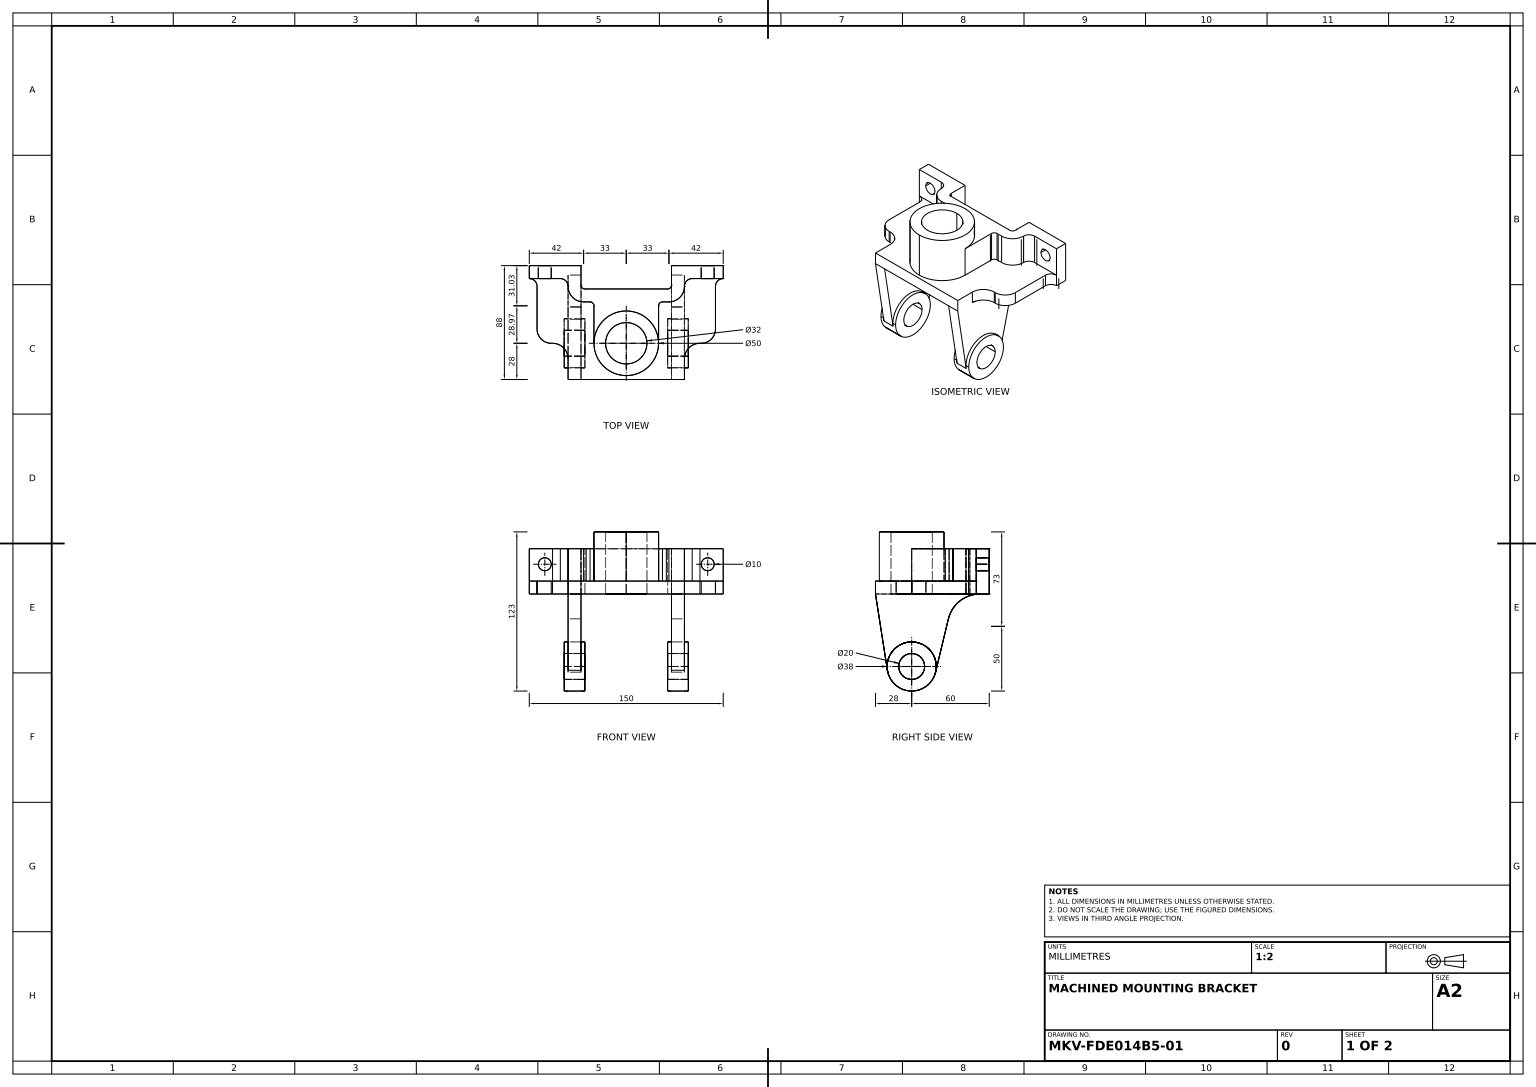
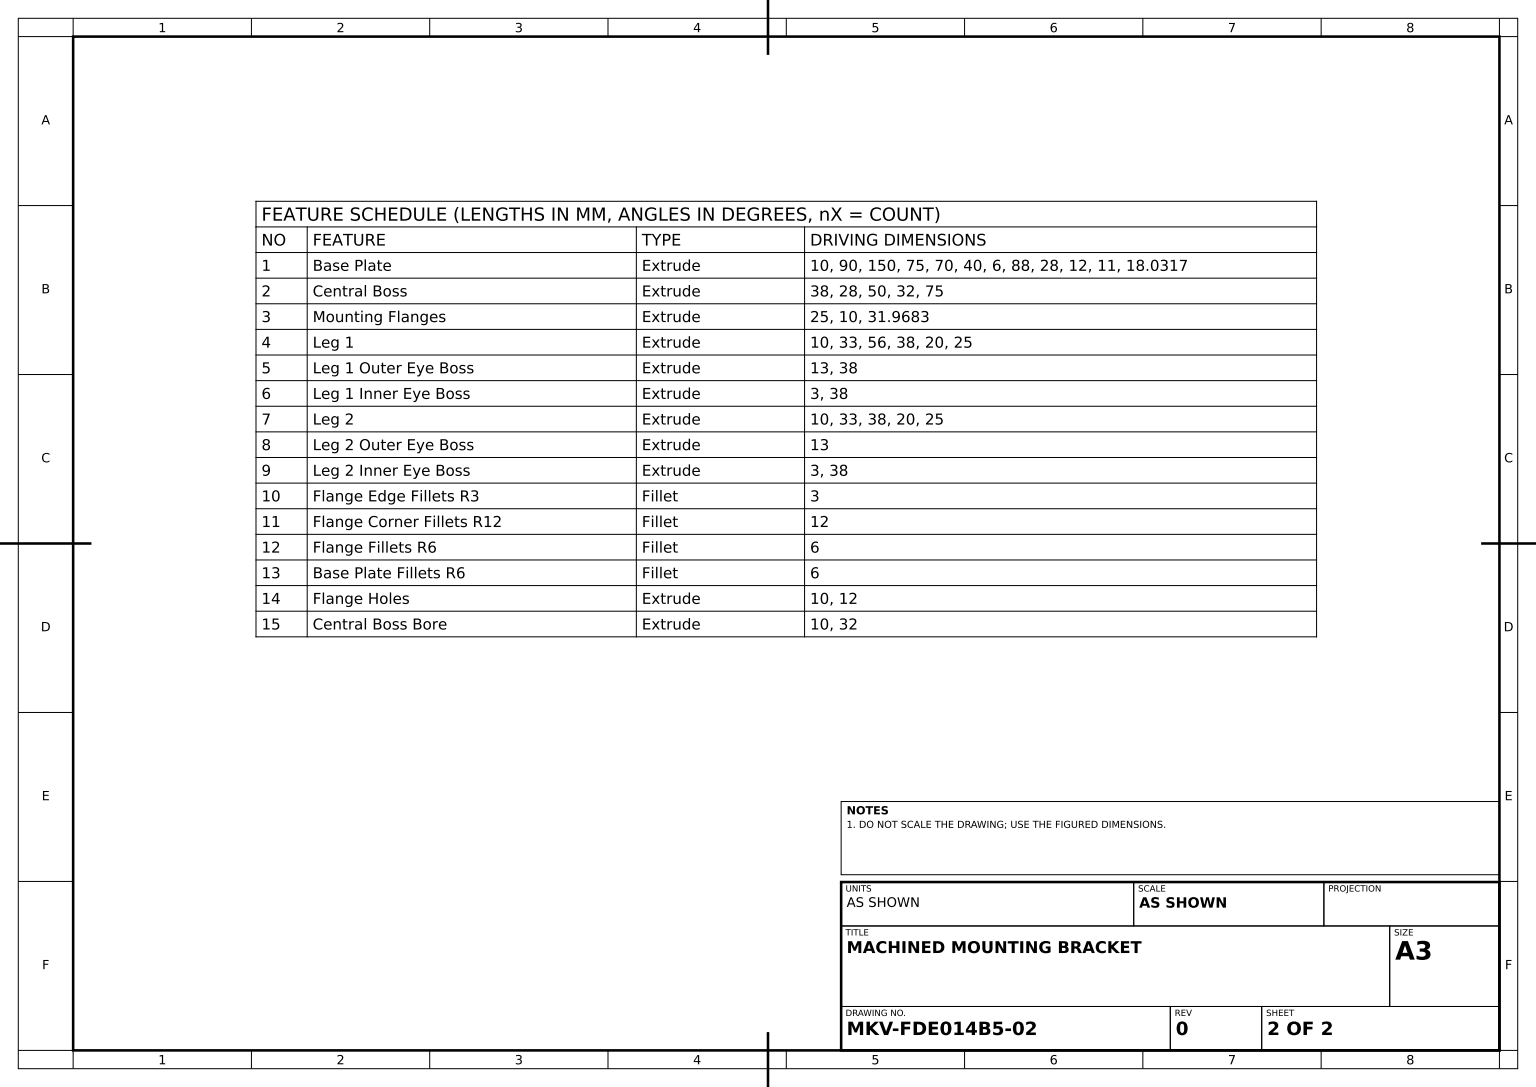
solid
v1 (-69,10,-39)
v2 (-58,10,-28)
e1 v1 v2 CIRCLE(AX(P(-58,10,-39),D(0,1,0),D(0,0,-1)),11)
v3 (-69,0,-39)
e2 v1 v3 LINE
v4 (-58,0,-28)
e3 v3 v4 CIRCLE(AX(P(-58,0,-39),D(0,1,0),D(0,0,-1)),11)
e4 v2 v4 LINE
face CYL(AX(P(-58,10,-39),D(0,-1,0),D(0,0,-1)),11) [-e1 e2 e3 -e4]
v5 (-51,35,-78)
v6 (-45,35,-72)
e5 v5 v6 CIRCLE(AX(P(-51,35,-72),D(0,-1,0),D(0,0,1)),6)
v7 (-51,10,-78)
e6 v7 v5 LINE
v8 (-45,10,-72)
e7 v8 v7 CIRCLE(AX(P(-51,10,-72),D(0,1,0),D(0,0,-1)),6)
e8 v6 v8 LINE
face CYL(AX(P(-51,35,-72),D(0,1,0),D(0,0,1)),6) rev [-e5 -e6 -e7 -e8]
v9 (32,35,-69.968306)
v10 (-32,35,-69.968306)
e9 v9 v10 LINE
v11 (32,0,-69.968306)
e10 v9 v11 LINE
v12 (-32,0,-69.968306)
e11 v11 v12 LINE
e12 v12 v10 LINE
face PLANE(AX(P(35,10,-69.968306),D(0,0,1),D(1,0,0))) rev [-e9 e10 e11 e12]
v13 (32,-56,-47)
v14 (35,-56,-47)
e13 v13 v14 LINE
v15 (32,-56,-9)
e14 v13 v15 CIRCLE(AX(P(32,-56,-28),D(1,0,0),D(0,0,-1)),19)
v16 (35,-56,-9)
e15 v15 v16 LINE
e16 v14 v16 CIRCLE(AX(P(35,-56,-28),D(1,0,0),D(0,0,-1)),19)
face CYL(AX(P(35,-56,-28),D(1,0,0),D(0,0,-1)),19) [-e13 e14 e15 -e16]
v17 (58,0,-28)
v18 (69,0,-39)
e17 v17 v18 CIRCLE(AX(P(58,0,-39),D(0,1,0),D(0,0,-1)),11)
v19 (69,10,-39)
e18 v19 v18 LINE
v20 (58,10,-28)
e19 v20 v19 CIRCLE(AX(P(58,10,-39),D(0,1,0),D(0,0,-1)),11)
e20 v20 v17 LINE
face CYL(AX(P(58,10,-39),D(0,-1,0),D(0,0,-1)),11) [e17 -e18 -e19 e20]
v21 (-25,35,-56.968306)
v22 (-25,35,-28)
e21 v21 v22 LINE
v23 (-25,10,-56.968306)
e22 v21 v23 LINE
v24 (-25,10,-28)
e23 v23 v24 LINE
e24 v22 v24 LINE
face PLANE(AX(P(-25,35,-28),D(1,0,0),D(0,0,-1))) rev [-e21 e22 e23 -e24]
v25 (68,23,-88)
v26 (58,23,-88)
e25 v25 v26 CIRCLE(AX(P(63,23,-88),D(0,0,-1),D(-1,0,0)),5)
e26 v26 v25 CIRCLE(AX(P(63,23,-88),D(0,0,-1),D(-1,0,0)),5)
v27 (75,0,-88)
v28 (35,0,-88)
e27 v27 v28 LINE
v29 (35,35,-88)
e28 v29 v28 LINE
v30 (75,35,-88)
e29 v30 v29 LINE
e30 v30 v27 LINE
face PLANE(AX(P(75,10,-88),D(0,0,1),D(1,0,0))) rev [-e25 -e26] [e27 -e28 -e29 e30]
v31 (75,35,-78)
e31 v31 v30 LINE
v32 (75,10,-78)
e32 v31 v32 LINE
v33 (75,0,-78)
e33 v32 v33 LINE
e34 v33 v27 LINE
face PLANE(AX(P(75,10,-78),D(-1,0,0),D(0,0,1))) rev [-e31 e32 e33 e34 -e30]
v34 (45,10,0)
v35 (45,0,0)
e35 v34 v35 LINE
v36 (-45,10,0)
e36 v36 v34 LINE
v37 (-45,0,0)
e37 v36 v37 LINE
v38 (-35,0,0)
e38 v37 v38 LINE
v39 (35,0,0)
e39 v38 v39 LINE
e40 v39 v35 LINE
face PLANE(AX(P(-45,10,0),D(0,0,-1),D(-1,0,0))) rev [-e35 -e36 e37 e38 e39 e40]
v40 (-33,35,-59.968306)
v41 (-28,35,-59.968306)
e41 v40 v41 LINE
v42 (-33,10,-59.968306)
e42 v40 v42 LINE
v43 (-28,10,-59.968306)
e43 v42 v43 LINE
e44 v43 v41 LINE
face PLANE(AX(P(-45,35,-59.968306),D(0,0,-1),D(-1,0,0))) rev [-e41 e42 e43 e44]
v44 (35,-60.439999,-46.473939)
v45 (35,-19.157895,-56.395619)
e45 v44 v45 LINE
e46 v44 v14 CIRCLE(AX(P(35,-56,-28),D(1,0,0),D(0,0,-1)),19)
v46 (35,-58.939212,-9.228718)
e47 v16 v46 CIRCLE(AX(P(35,-56,-28),D(1,0,0),D(0,0,-1)),19)
e48 v39 v46 LINE
v47 (35,0,-72.968306)
e49 v47 v39 LINE
v48 (35,35,-72.968306)
e50 v47 v48 LINE
e51 v29 v48 LINE
v49 (35,0,-80.703433)
e52 v28 v49 LINE
e53 v45 v49 CIRCLE(AX(P(35,-25,-80.703433),D(-1,0,0),D(0,0,-1)),25)
face PLANE(AX(P(35,10,-88),D(1,0,0),D(0,0,-1))) rev [-e45 e46 e16 e47 -e48 -e49 e50 -e51 e28 e52 -e53]
v50 (-48,-56,-18)
v51 (-48,-56,-38)
e54 v50 v51 CIRCLE(AX(P(-48,-56,-28),D(-1,0,0),D(0,0,1)),10)
e55 v51 v50 CIRCLE(AX(P(-48,-56,-28),D(-1,0,0),D(0,0,1)),10)
v52 (-48,-56,-47)
v53 (-48,-56,-9)
e56 v52 v53 CIRCLE(AX(P(-48,-56,-28),D(-1,0,0),D(0,0,1)),19)
e57 v53 v52 CIRCLE(AX(P(-48,-56,-28),D(-1,0,0),D(0,0,1)),19)
face PLANE(AX(P(-48,-56,-28),D(-1,0,0),D(0,0,1))) [-e54 -e55] [e56 e57]
v54 (51,35,-78)
v55 (51,10,-78)
e58 v54 v55 LINE
v56 (45,35,-72)
e59 v56 v54 CIRCLE(AX(P(51,35,-72),D(0,-1,0),D(0,0,1)),6)
v57 (45,10,-72)
e60 v57 v56 LINE
e61 v55 v57 CIRCLE(AX(P(51,10,-72),D(0,1,0),D(0,0,-1)),6)
face CYL(AX(P(51,10,-72),D(0,1,0),D(0,0,1)),6) rev [-e58 -e59 -e60 -e61]
v58 (-45,-58.939212,-9.228718)
e62 v58 v37 LINE
v59 (-35,-58.939212,-9.228718)
e63 v59 v58 LINE
e64 v59 v38 LINE
face PLANE(AX(P(-35,0,0),D(0,-0.154695393,0.987962214),D(0,-0.987962214,-0.154695393))) [-e62 -e63 e64 -e38]
v60 (-68,23,-88)
v61 (-58,23,-88)
e65 v60 v61 CIRCLE(AX(P(-63,23,-88),D(0,0,-1),D(-1,0,0)),5)
v62 (-58,23,-78)
e66 v62 v61 LINE
v63 (-68,23,-78)
e67 v63 v62 CIRCLE(AX(P(-63,23,-78),D(0,0,-1),D(-1,0,0)),5)
e68 v63 v60 LINE
face CYL(AX(P(-63,23,-78),D(0,0,-1),D(-1,0,0)),5) rev [e65 -e66 -e67 e68]
v64 (-45,35,-71.968306)
e69 v6 v64 LINE
v65 (-45,10,-71.968306)
e70 v8 v65 LINE
e71 v65 v64 LINE
face PLANE(AX(P(-45,35,-78),D(1,0,0),D(0,0,-1))) rev [-e69 e8 e70 e71]
v66 (68,23,-78)
e72 v66 v25 LINE
v67 (58,23,-78)
e73 v67 v66 CIRCLE(AX(P(63,23,-78),D(0,0,-1),D(-1,0,0)),5)
e74 v67 v26 LINE
face CYL(AX(P(63,23,-78),D(0,0,-1),D(-1,0,0)),5) rev [-e72 -e73 e74 e26]
v68 (32,-56,-38)
v69 (32,-56,-18)
e75 v68 v69 CIRCLE(AX(P(32,-56,-28),D(1,0,0),D(0,0,-1)),10)
v70 (48,-56,-38)
e76 v68 v70 LINE
v71 (48,-56,-18)
e77 v70 v71 CIRCLE(AX(P(48,-56,-28),D(1,0,0),D(0,0,-1)),10)
e78 v69 v71 LINE
face CYL(AX(P(35,-56,-28),D(1,0,0),D(0,0,-1)),10) rev [-e75 e76 e77 -e78]
v72 (69,10,-72)
e79 v19 v72 LINE
e80 v72 v32 CIRCLE(AX(P(75,10,-72),D(0,-1,0),D(0,0,-1)),6)
e81 v55 v32 LINE
v73 (45,10,-71.968306)
e82 v73 v57 LINE
v74 (33,10,-59.968306)
e83 v73 v74 CIRCLE(AX(P(33,10,-71.968306),D(0,-1,0),D(0,0,-1)),12)
v75 (28,10,-59.968306)
e84 v75 v74 LINE
v76 (25,10,-56.968306)
e85 v75 v76 CIRCLE(AX(P(28,10,-56.968306),D(0,1,0),D(0,0,-1)),3)
v77 (25,10,-28)
e86 v77 v76 LINE
v78 (0,10,-3)
e87 v78 v77 CIRCLE(AX(P(0,10,-28),D(0,1,0),D(0,0,-1)),25)
e88 v24 v78 CIRCLE(AX(P(0,10,-28),D(0,1,0),D(0,0,-1)),25)
e89 v23 v43 CIRCLE(AX(P(-28,10,-56.968306),D(0,1,0),D(0,0,-1)),3)
e90 v42 v65 CIRCLE(AX(P(-33,10,-71.968306),D(0,-1,0),D(0,0,-1)),12)
v79 (-75,10,-78)
e91 v79 v7 LINE
v80 (-69,10,-72)
e92 v79 v80 CIRCLE(AX(P(-75,10,-72),D(0,-1,0),D(0,0,-1)),6)
e93 v80 v1 LINE
v81 (-57,10,-28)
e94 v2 v81 LINE
v82 (-45,10,-16)
e95 v81 v82 CIRCLE(AX(P(-57,10,-16),D(0,-1,0),D(0,0,1)),12)
e96 v82 v36 LINE
v83 (45,10,-16)
e97 v34 v83 LINE
v84 (57,10,-28)
e98 v83 v84 CIRCLE(AX(P(57,10,-16),D(0,-1,0),D(0,0,1)),12)
e99 v84 v20 LINE
face PLANE(AX(P(-58,10,-39),D(0,-1,0),D(0,0,-1))) rev [e19 e79 e80 -e81 e61 -e82 e83 -e84 e85 -e86 -e87 -e88 -e23 e89 -e43 e90 -e70 e7 -e91 e92 e93 e1 e94 e95 e96 e36 e97 e98 e99]
v85 (-32,-56,-47)
v86 (-32,-56,-9)
e100 v85 v86 CIRCLE(AX(P(-32,-56,-28),D(-1,0,0),D(0,0,1)),19)
v87 (-35,-56,-9)
e101 v86 v87 LINE
e102 v59 v87 CIRCLE(AX(P(-35,-56,-28),D(-1,0,0),D(0,0,1)),19)
v88 (-45,-56,-9)
e103 v58 v88 CIRCLE(AX(P(-45,-56,-28),D(-1,0,0),D(0,0,1)),19)
e104 v88 v53 LINE
v89 (-45,-56,-47)
e105 v89 v52 LINE
v90 (-45,-60.439999,-46.473939)
e106 v89 v90 CIRCLE(AX(P(-45,-56,-28),D(-1,0,0),D(0,0,1)),19)
v91 (-35,-60.439999,-46.473939)
e107 v91 v90 LINE
v92 (-35,-56,-47)
e108 v92 v91 CIRCLE(AX(P(-35,-56,-28),D(-1,0,0),D(0,0,1)),19)
e109 v85 v92 LINE
face CYL(AX(P(-35,-56,-28),D(-1,0,0),D(0,0,1)),19) [e100 e101 -e102 e63 e103 e104 -e56 -e105 e106 -e107 -e108 -e109]
v93 (69,0,-72)
e110 v33 v93 CIRCLE(AX(P(75,0,-72),D(0,1,0),D(0,0,-1)),6)
e111 v18 v93 LINE
v94 (57,0,-28)
e112 v94 v17 LINE
v95 (45,0,-16)
e113 v95 v94 CIRCLE(AX(P(57,0,-16),D(0,-1,0),D(0,0,1)),12)
v96 (45,0,-80.703433)
e114 v96 v95 LINE
e115 v49 v96 LINE
face PLANE(AX(P(-58,0,-39),D(0,-1,0),D(0,0,-1))) [-e34 e110 -e111 -e17 -e112 -e113 -e114 -e115 -e52 -e27]
v97 (-75,35,-88)
v98 (-75,35,-78)
e116 v97 v98 LINE
v99 (-75,0,-88)
e117 v97 v99 LINE
v100 (-75,0,-78)
e118 v99 v100 LINE
e119 v79 v100 LINE
e120 v98 v79 LINE
face PLANE(AX(P(-75,10,-88),D(1,0,0),D(0,0,-1))) rev [-e116 e117 e118 -e119 -e120]
v101 (25,35,-56.968306)
v102 (28,35,-59.968306)
e121 v101 v102 CIRCLE(AX(P(28,35,-56.968306),D(0,-1,0),D(0,0,1)),3)
e122 v76 v101 LINE
e123 v102 v75 LINE
face CYL(AX(P(28,35,-56.968306),D(0,1,0),D(0,0,1)),3) rev [-e121 -e122 -e85 -e123]
e124 v93 v72 LINE
face PLANE(AX(P(69,10,-39),D(-1,0,0),D(0,0,1))) rev [-e79 e18 e111 e124]
v103 (25,35,-28)
e125 v103 v101 LINE
e126 v103 v77 LINE
face PLANE(AX(P(25,35,-28),D(-1,0,0),D(0,0,1))) rev [e122 -e125 e126 e86]
v104 (48,-56,-9)
v105 (48,-56,-47)
e127 v104 v105 CIRCLE(AX(P(48,-56,-28),D(1,0,0),D(0,0,-1)),19)
e128 v105 v104 CIRCLE(AX(P(48,-56,-28),D(1,0,0),D(0,0,-1)),19)
e129 v71 v70 CIRCLE(AX(P(48,-56,-28),D(1,0,0),D(0,0,-1)),10)
face PLANE(AX(P(48,-56,-28),D(1,0,0),D(0,0,-1))) [e127 e128] [-e129 -e77]
v106 (-32,-56,-38)
e130 v106 v51 LINE
v107 (-32,-56,-18)
e131 v107 v50 LINE
e132 v106 v107 CIRCLE(AX(P(-32,-56,-28),D(-1,0,0),D(0,0,1)),10)
face CYL(AX(P(-35,-56,-28),D(-1,0,0),D(0,0,1)),10) rev [e130 e55 -e131 -e132]
e133 v86 v85 CIRCLE(AX(P(-32,-56,-28),D(-1,0,0),D(0,0,1)),19)
e134 v87 v92 CIRCLE(AX(P(-35,-56,-28),D(-1,0,0),D(0,0,1)),19)
face CYL(AX(P(-35,-56,-28),D(-1,0,0),D(0,0,1)),19) [e133 e109 -e134 -e101]
v108 (45,-60.439999,-46.473939)
e135 v44 v108 LINE
v109 (45,-56,-47)
e136 v108 v109 CIRCLE(AX(P(45,-56,-28),D(1,0,0),D(0,0,-1)),19)
e137 v109 v105 LINE
v110 (45,-56,-9)
e138 v110 v104 LINE
v111 (45,-58.939212,-9.228718)
e139 v110 v111 CIRCLE(AX(P(45,-56,-28),D(1,0,0),D(0,0,-1)),19)
e140 v46 v111 LINE
e141 v15 v13 CIRCLE(AX(P(32,-56,-28),D(1,0,0),D(0,0,-1)),19)
face CYL(AX(P(35,-56,-28),D(1,0,0),D(0,0,-1)),19) [-e46 e135 e136 e137 -e127 -e138 e139 -e140 -e47 -e15 e141 e13]
e142 v11 v47 CIRCLE(AX(P(32,0,-72.968306),D(0,1,0),D(0,0,-1)),3)
e143 v48 v9 CIRCLE(AX(P(32,35,-72.968306),D(0,-1,0),D(0,0,1)),3)
face CYL(AX(P(32,10,-72.968306),D(0,1,0),D(0,0,1)),3) rev [-e50 -e142 -e10 -e143]
v112 (-69,0,-72)
e144 v112 v100 CIRCLE(AX(P(-75,0,-72),D(0,1,0),D(0,0,-1)),6)
v113 (-35,0,-88)
e145 v113 v99 LINE
v114 (-35,0,-80.703433)
e146 v114 v113 LINE
v115 (-45,0,-80.703433)
e147 v114 v115 LINE
v116 (-45,0,-16)
e148 v116 v115 LINE
v117 (-57,0,-28)
e149 v117 v116 CIRCLE(AX(P(-57,0,-16),D(0,-1,0),D(0,0,1)),12)
e150 v4 v117 LINE
e151 v112 v3 LINE
face PLANE(AX(P(-58,0,-39),D(0,-1,0),D(0,0,-1))) [e144 -e118 -e145 -e146 e147 -e148 -e149 -e150 -e3 -e151]
e152 v82 v116 LINE
v118 (-45,-19.157895,-56.395619)
e153 v115 v118 CIRCLE(AX(P(-45,-25,-80.703433),D(1,0,0),D(0,0,-1)),25)
e154 v118 v90 LINE
e155 v88 v89 CIRCLE(AX(P(-45,-56,-28),D(-1,0,0),D(0,0,1)),19)
face PLANE(AX(P(-45,10,-16),D(1,0,0),D(0,0,-1))) rev [-e103 e62 -e37 -e96 e152 e148 e153 e154 -e106 -e155]
v119 (-35,35,-88)
e156 v119 v113 LINE
v120 (-35,35,-72.968306)
e157 v120 v119 LINE
v121 (-35,0,-72.968306)
e158 v120 v121 LINE
e159 v38 v121 LINE
v122 (-35,-19.157895,-56.395619)
e160 v122 v91 LINE
e161 v114 v122 CIRCLE(AX(P(-35,-25,-80.703433),D(1,0,0),D(0,0,-1)),25)
face PLANE(AX(P(-35,10,-69.968306),D(-1,0,0),D(0,0,1))) rev [e146 -e156 -e157 e158 -e159 -e64 e102 e134 e108 -e160 -e161]
face CYL(AX(P(75,10,-72),D(0,1,0),D(0,0,1)),6) rev [-e124 -e110 -e33 -e80]
e162 v54 v31 LINE
e163 v66 v67 CIRCLE(AX(P(63,23,-78),D(0,0,-1),D(-1,0,0)),5)
face PLANE(AX(P(69,10,-78),D(0,0,-1),D(-1,0,0))) rev [e58 e81 -e32 -e162] [e163 e73]
e164 v109 v110 CIRCLE(AX(P(45,-56,-28),D(1,0,0),D(0,0,-1)),19)
face CYL(AX(P(35,-56,-28),D(1,0,0),D(0,0,-1)),19) [e164 e138 -e128 -e137]
e165 v84 v94 LINE
face PLANE(AX(P(57,10,-28),D(0,0,-1),D(-1,0,0))) rev [-e20 -e99 e165 e112]
face CYL(AX(P(63,23,-78),D(0,0,-1),D(-1,0,0)),5) rev [-e74 -e163 e72 e25]
e166 v80 v112 LINE
face PLANE(AX(P(-69,10,-78),D(1,0,0),D(0,0,-1))) rev [e151 -e2 -e93 e166]
e167 v81 v117 LINE
face CYL(AX(P(-57,10,-16),D(0,-1,0),D(0,0,-1)),12) rev [e167 e149 -e152 -e95]
e168 v41 v21 CIRCLE(AX(P(-28,35,-56.968306),D(0,-1,0),D(0,0,1)),3)
face CYL(AX(P(-28,35,-56.968306),D(0,1,0),D(0,0,1)),3) rev [-e44 -e89 -e22 -e168]
e169 v107 v106 CIRCLE(AX(P(-32,-56,-28),D(-1,0,0),D(0,0,1)),10)
face PLANE(AX(P(-32,-56,-28),D(-1,0,0),D(0,0,1))) rev [-e133 -e100] [e169 e132]
e170 v122 v118 LINE
face PLANE(AX(P(-35,-19.157895,-56.395619),D(0,-0.233684184,-0.972312554),D(0,0.972312554,-0.233684184))) [-e170 e160 e107 -e154]
e171 v64 v40 CIRCLE(AX(P(-33,35,-71.968306),D(0,1,0),D(0,0,1)),12)
face CYL(AX(P(-33,35,-71.968306),D(0,-1,0),D(0,0,-1)),12) [-e90 -e42 -e171 -e71]
e172 v10 v120 CIRCLE(AX(P(-32,35,-72.968306),D(0,-1,0),D(0,0,1)),3)
e173 v121 v12 CIRCLE(AX(P(-32,0,-72.968306),D(0,1,0),D(0,0,-1)),3)
face CYL(AX(P(-32,10,-72.968306),D(0,1,0),D(0,0,1)),3) rev [-e158 -e172 -e12 -e173]
e174 v69 v68 CIRCLE(AX(P(32,-56,-28),D(1,0,0),D(0,0,-1)),10)
face PLANE(AX(P(32,-56,-28),D(1,0,0),D(0,0,-1))) rev [-e14 -e141] [e75 e174]
e175 v83 v95 LINE
face CYL(AX(P(57,10,-16),D(0,-1,0),D(0,0,-1)),12) rev [e175 e113 -e165 -e98]
face CYL(AX(P(-75,10,-72),D(0,1,0),D(0,0,1)),6) rev [-e92 e119 -e144 -e166]
v123 (0,35,-53)
e176 v22 v123 CIRCLE(AX(P(0,35,-28),D(0,-1,0),D(0,0,1)),25)
v124 (0,48,-3)
e177 v124 v78 LINE
v125 (0,48,-53)
e178 v125 v124 CIRCLE(AX(P(0,48,-28),D(0,1,0),D(0,0,1)),25)
e179 v125 v123 LINE
face CYL(AX(P(0,48,-28),D(0,-1,0),D(0,0,-1)),25) [-e176 e24 e88 -e177 -e178 e179]
face CYL(AX(P(-35,-25,-80.703433),D(-1,0,0),D(0,0,1)),25) rev [-e153 -e147 e161 e170]
v126 (45,-19.157895,-56.395619)
e180 v126 v96 CIRCLE(AX(P(45,-25,-80.703433),D(-1,0,0),D(0,0,-1)),25)
e181 v45 v126 LINE
face CYL(AX(P(35,-25,-80.703433),D(1,0,0),D(0,0,-1)),25) rev [-e180 -e181 e53 e115]
face CYL(AX(P(35,-56,-28),D(1,0,0),D(0,0,-1)),10) rev [-e174 e78 e129 -e76]
e182 v61 v60 CIRCLE(AX(P(-63,23,-88),D(0,0,-1),D(-1,0,0)),5)
e183 v62 v63 CIRCLE(AX(P(-63,23,-78),D(0,0,-1),D(-1,0,0)),5)
face CYL(AX(P(-63,23,-78),D(0,0,-1),D(-1,0,0)),5) rev [e182 -e68 -e183 e66]
v127 (33,35,-59.968306)
e184 v74 v127 LINE
e185 v102 v127 LINE
face PLANE(AX(P(45,35,-59.968306),D(0,0,-1),D(-1,0,0))) rev [e184 -e185 e123 e84]
e186 v98 v5 LINE
face PLANE(AX(P(-75,10,-78),D(0,0,-1),D(-1,0,0))) rev [e183 e67] [e91 e6 -e186 e120]
e187 v123 v103 CIRCLE(AX(P(0,35,-28),D(0,-1,0),D(0,0,1)),25)
v128 (45,35,-71.968306)
e188 v127 v128 CIRCLE(AX(P(33,35,-71.968306),D(0,1,0),D(0,0,1)),12)
e189 v128 v56 LINE
e190 v119 v97 LINE
face PLANE(AX(P(0,35,-28),D(0,1,0),D(0,0,1))) [e116 e186 e5 e69 e171 e41 e168 e21 e176 e187 e125 e121 e185 e188 e189 e59 e162 e31 e29 e51 e143 e9 e172 e157 e190]
e191 v108 v126 LINE
e192 v35 v111 LINE
face PLANE(AX(P(45,10,0),D(-1,0,0),D(0,0,1))) rev [-e139 -e164 -e136 e191 e180 e114 -e175 -e97 e35 e192]
e193 v128 v73 LINE
face CYL(AX(P(33,35,-71.968306),D(0,-1,0),D(0,0,-1)),12) [-e188 -e184 -e83 -e193]
face CYL(AX(P(-35,-56,-28),D(-1,0,0),D(0,0,1)),10) rev [-e130 -e169 e131 e54]
v129 (0,48,-44)
v130 (0,48,-12)
e194 v129 v130 CIRCLE(AX(P(0,48,-28),D(0,1,0),D(0,0,1)),16)
e195 v130 v129 CIRCLE(AX(P(0,48,-28),D(0,1,0),D(0,0,1)),16)
e196 v124 v125 CIRCLE(AX(P(0,48,-28),D(0,1,0),D(0,0,1)),25)
face PLANE(AX(P(0,48,-28),D(0,1,0),D(0,0,1))) [-e194 -e195] [e178 e196]
v131 (0,0,-12)
e197 v130 v131 LINE
v132 (0,0,-44)
e198 v132 v131 CIRCLE(AX(P(0,0,-28),D(0,1,0),D(0,0,1)),16)
e199 v129 v132 LINE
face CYL(AX(P(0,48,-28),D(0,-1,0),D(0,0,-1)),16) rev [e197 -e198 -e199 e194]
e200 v131 v132 CIRCLE(AX(P(0,0,-28),D(0,1,0),D(0,0,1)),16)
face CYL(AX(P(0,48,-28),D(0,-1,0),D(0,0,-1)),16) rev [e199 -e200 -e197 e195]
face PLANE(AX(P(-58,10,-28),D(0,0,-1),D(-1,0,0))) rev [e150 -e167 -e94 e4]
face PLANE(AX(P(-58,0,-39),D(0,-1,0),D(0,0,-1))) [e173 -e11 e142 e49 -e39 e159] [e200 e198]
face PLANE(AX(P(-35,10,-88),D(0,0,1),D(1,0,0))) rev [e145 -e117 -e190 e156] [-e182 -e65]
face CYL(AX(P(0,48,-28),D(0,-1,0),D(0,0,-1)),25) [e177 e87 -e126 -e187 -e179 -e196]
face PLANE(AX(P(35,-19.157895,-56.395619),D(0,-0.233684184,-0.972312554),D(0,0.972312554,-0.233684184))) [-e191 -e135 e45 e181]
face PLANE(AX(P(35,0,0),D(0,-0.154695393,0.987962214),D(0,-0.987962214,-0.154695393))) [-e192 -e40 e48 e140]
face CYL(AX(P(-35,-56,-28),D(-1,0,0),D(0,0,1)),19) [-e57 -e104 e155 e105]
face PLANE(AX(P(45,35,-78),D(-1,0,0),D(0,0,1))) rev [-e189 e193 e82 e60]
